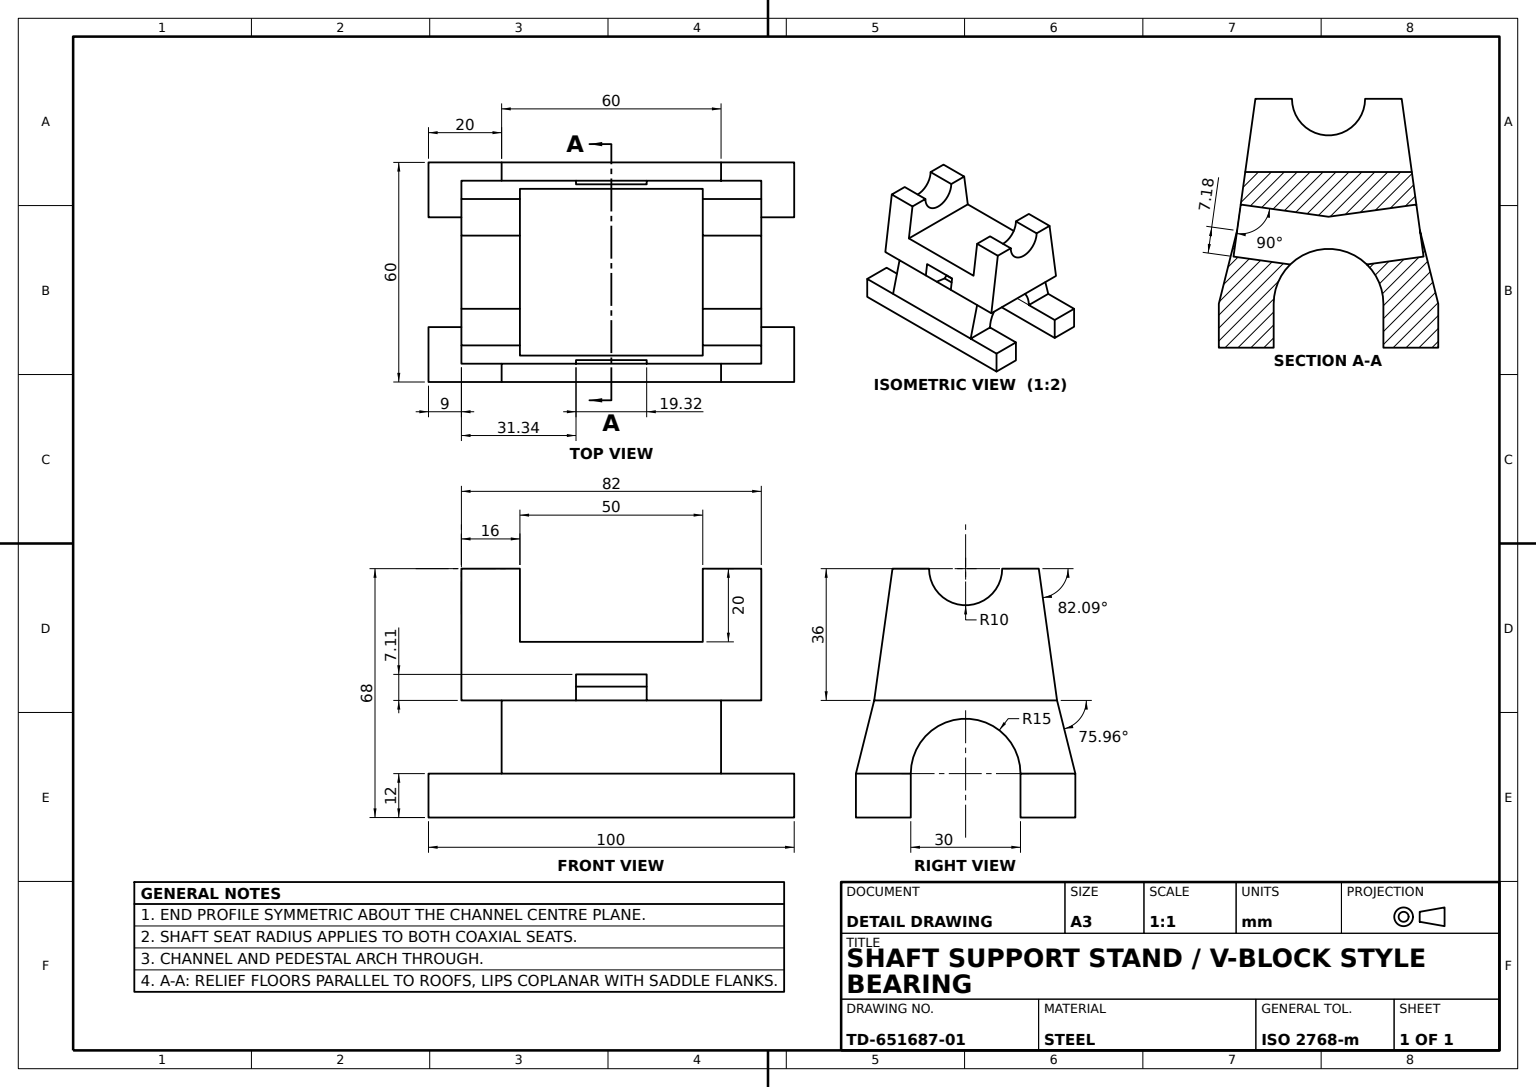
ISO-10303-21;
HEADER;
FILE_DESCRIPTION((''),'2;1');
FILE_NAME('','',(''),(''),'','','');
FILE_SCHEMA(('AUTOMOTIVE_DESIGN'));
ENDSEC;
DATA;
#1=APPLICATION_CONTEXT('');
#2=PRODUCT_CONTEXT('',#1,'mechanical');
#3=PRODUCT('','','',(#2));
#4=PRODUCT_DEFINITION_FORMATION('','',#3);
#5=PRODUCT_DEFINITION_CONTEXT('',#1,'design');
#6=PRODUCT_DEFINITION('','',#4,#5);
#7=PRODUCT_DEFINITION_SHAPE('','',#6);
#8=(LENGTH_UNIT()NAMED_UNIT(*)SI_UNIT(.MILLI.,.METRE.));
#9=(NAMED_UNIT(*)PLANE_ANGLE_UNIT()SI_UNIT($,.RADIAN.));
#10=(NAMED_UNIT(*)SI_UNIT($,.STERADIAN.)SOLID_ANGLE_UNIT());
#11=UNCERTAINTY_MEASURE_WITH_UNIT(LENGTH_MEASURE(1.E-05),#8,'distance_accuracy_value','');
#12=(GEOMETRIC_REPRESENTATION_CONTEXT(3)GLOBAL_UNCERTAINTY_ASSIGNED_CONTEXT((#11))GLOBAL_UNIT_ASSIGNED_CONTEXT((#8,#9,#10))REPRESENTATION_CONTEXT('',''));
#13=CARTESIAN_POINT('',(-15.,0.,-100.));
#14=VERTEX_POINT('',#13);
#15=CARTESIAN_POINT('',(-15.,0.,0.));
#16=VERTEX_POINT('',#15);
#17=DIRECTION('',(0.,0.,1.));
#18=VECTOR('',#17,1000.);
#19=LINE('',#15,#18);
#20=EDGE_CURVE('',#14,#16,#19,.T.);
#21=ORIENTED_EDGE('',*,*,#20,.T.);
#22=CARTESIAN_POINT('',(-30.,0.,0.));
#23=VERTEX_POINT('',#22);
#24=CARTESIAN_POINT('',(0.,0.,0.));
#25=DIRECTION('',(1.,0.,0.));
#26=VECTOR('',#25,1000.);
#27=LINE('',#24,#26);
#28=EDGE_CURVE('',#23,#16,#27,.T.);
#29=ORIENTED_EDGE('',*,*,#28,.F.);
#30=CARTESIAN_POINT('',(-30.,0.,-100.));
#31=VERTEX_POINT('',#30);
#32=LINE('',#30,#18);
#33=EDGE_CURVE('',#31,#23,#32,.T.);
#34=ORIENTED_EDGE('',*,*,#33,.F.);
#35=CARTESIAN_POINT('',(30.,0.,-100.));
#36=DIRECTION('',(-1.,0.,0.));
#37=VECTOR('',#36,1000.);
#38=LINE('',#35,#37);
#39=EDGE_CURVE('',#14,#31,#38,.T.);
#40=ORIENTED_EDGE('',*,*,#39,.F.);
#41=EDGE_LOOP('',(#21,#29,#34,#40));
#42=FACE_OUTER_BOUND('',#41,.T.);
#43=DIRECTION('',(0.,1.,0.));
#44=AXIS2_PLACEMENT_3D('',#24,#43,#17);
#45=PLANE('',#44);
#46=ADVANCED_FACE('',(#42),#45,.F.);
#47=CARTESIAN_POINT('',(-25.,32.,-80.));
#48=VERTEX_POINT('',#47);
#49=CARTESIAN_POINT('',(-30.,12.,-80.));
#50=VERTEX_POINT('',#49);
#51=DIRECTION('',(-0.242535625,-0.9701425,0.));
#52=VECTOR('',#51,1000.);
#53=LINE('',#47,#52);
#54=EDGE_CURVE('',#48,#50,#53,.T.);
#55=ORIENTED_EDGE('',*,*,#54,.T.);
#56=CARTESIAN_POINT('',(-30.,12.,-20.));
#57=VERTEX_POINT('',#56);
#58=LINE('',#49,#18);
#59=EDGE_CURVE('',#50,#57,#58,.T.);
#60=ORIENTED_EDGE('',*,*,#59,.T.);
#61=CARTESIAN_POINT('',(-25.,32.,-20.));
#62=VERTEX_POINT('',#61);
#63=LINE('',#61,#52);
#64=EDGE_CURVE('',#62,#57,#63,.T.);
#65=ORIENTED_EDGE('',*,*,#64,.F.);
#66=CARTESIAN_POINT('',(-25.,32.,-40.337526));
#67=VERTEX_POINT('',#66);
#68=LINE('',#47,#18);
#69=EDGE_CURVE('',#67,#62,#68,.T.);
#70=ORIENTED_EDGE('',*,*,#69,.F.);
#71=CARTESIAN_POINT('',(-25.,32.,-59.662474));
#72=VERTEX_POINT('',#71);
#73=EDGE_CURVE('',#72,#67,#68,.T.);
#74=ORIENTED_EDGE('',*,*,#73,.F.);
#75=EDGE_CURVE('',#48,#72,#68,.T.);
#76=ORIENTED_EDGE('',*,*,#75,.F.);
#77=EDGE_LOOP('',(#55,#60,#65,#70,#74,#76));
#78=FACE_OUTER_BOUND('',#77,.T.);
#79=DIRECTION('',(-0.9701425,0.242535625,0.));
#80=AXIS2_PLACEMENT_3D('',#47,#79,#51);
#81=PLANE('',#80);
#82=ADVANCED_FACE('',(#78),#81,.T.);
#83=CARTESIAN_POINT('',(-30.,12.,0.));
#84=VERTEX_POINT('',#83);
#85=CARTESIAN_POINT('',(-15.,12.,0.));
#86=VERTEX_POINT('',#85);
#87=LINE('',#83,#26);
#88=EDGE_CURVE('',#84,#86,#87,.T.);
#89=ORIENTED_EDGE('',*,*,#88,.T.);
#90=CARTESIAN_POINT('',(-15.,12.,-20.));
#91=VERTEX_POINT('',#90);
#92=CARTESIAN_POINT('',(-15.,12.,-100.));
#93=LINE('',#92,#18);
#94=EDGE_CURVE('',#91,#86,#93,.T.);
#95=ORIENTED_EDGE('',*,*,#94,.F.);
#96=LINE('',#56,#26);
#97=EDGE_CURVE('',#57,#91,#96,.T.);
#98=ORIENTED_EDGE('',*,*,#97,.F.);
#99=CARTESIAN_POINT('',(-30.,12.,-100.));
#100=LINE('',#99,#18);
#101=EDGE_CURVE('',#57,#84,#100,.T.);
#102=ORIENTED_EDGE('',*,*,#101,.T.);
#103=EDGE_LOOP('',(#89,#95,#98,#102));
#104=FACE_OUTER_BOUND('',#103,.T.);
#105=CARTESIAN_POINT('',(0.,12.,0.));
#106=AXIS2_PLACEMENT_3D('',#105,#43,#17);
#107=PLANE('',#106);
#108=ADVANCED_FACE('',(#104),#107,.T.);
#109=CARTESIAN_POINT('',(-10.,68.,-75.));
#110=VERTEX_POINT('',#109);
#111=CARTESIAN_POINT('',(-20.,68.,-75.));
#112=VERTEX_POINT('',#111);
#113=LINE('',#111,#37);
#114=EDGE_CURVE('',#110,#112,#113,.T.);
#115=ORIENTED_EDGE('',*,*,#114,.T.);
#116=CARTESIAN_POINT('',(-22.777778,48.,-75.));
#117=VERTEX_POINT('',#116);
#118=DIRECTION('',(-0.137568371,-0.990492273,0.));
#119=VECTOR('',#118,1000.);
#120=LINE('',#111,#119);
#121=EDGE_CURVE('',#112,#117,#120,.T.);
#122=ORIENTED_EDGE('',*,*,#121,.T.);
#123=CARTESIAN_POINT('',(22.777778,48.,-75.));
#124=VERTEX_POINT('',#123);
#125=CARTESIAN_POINT('',(20.,48.,-75.));
#126=LINE('',#125,#37);
#127=EDGE_CURVE('',#124,#117,#126,.T.);
#128=ORIENTED_EDGE('',*,*,#127,.F.);
#129=CARTESIAN_POINT('',(20.,68.,-75.));
#130=VERTEX_POINT('',#129);
#131=DIRECTION('',(-0.137568371,0.990492273,0.));
#132=VECTOR('',#131,1000.);
#133=LINE('',#129,#132);
#134=EDGE_CURVE('',#124,#130,#133,.T.);
#135=ORIENTED_EDGE('',*,*,#134,.T.);
#136=CARTESIAN_POINT('',(10.,68.,-75.));
#137=VERTEX_POINT('',#136);
#138=EDGE_CURVE('',#130,#137,#113,.T.);
#139=ORIENTED_EDGE('',*,*,#138,.T.);
#140=CARTESIAN_POINT('',(0.,68.,-75.));
#141=DIRECTION('',(0.,0.,-1.));
#142=AXIS2_PLACEMENT_3D('',#140,#141,#36);
#143=CIRCLE('',#142,10.);
#144=EDGE_CURVE('',#137,#110,#143,.T.);
#145=ORIENTED_EDGE('',*,*,#144,.T.);
#146=EDGE_LOOP('',(#115,#122,#128,#135,#139,#145));
#147=FACE_OUTER_BOUND('',#146,.T.);
#148=CARTESIAN_POINT('',(-20.,48.,-75.));
#149=AXIS2_PLACEMENT_3D('',#148,#141,#36);
#150=PLANE('',#149);
#151=ADVANCED_FACE('',(#147),#150,.F.);
#152=CARTESIAN_POINT('',(-25.987343,24.891129,-59.662474));
#153=VERTEX_POINT('',#152);
#154=DIRECTION('',(0.137568371,0.990492273,0.));
#155=VECTOR('',#154,1000.);
#156=LINE('',#152,#155);
#157=EDGE_CURVE('',#153,#72,#156,.T.);
#158=ORIENTED_EDGE('',*,*,#157,.F.);
#159=CARTESIAN_POINT('',(-10.474958,22.736632,-59.662474));
#160=VERTEX_POINT('',#159);
#161=CARTESIAN_POINT('',(1.746441,21.039215,-59.662474));
#162=DIRECTION('',(-0.990492273,0.137568371,0.));
#163=VECTOR('',#162,1000.);
#164=LINE('',#161,#163);
#165=EDGE_CURVE('',#160,#153,#164,.T.);
#166=ORIENTED_EDGE('',*,*,#165,.F.);
#167=CARTESIAN_POINT('',(10.474958,22.736632,-59.662474));
#168=VERTEX_POINT('',#167);
#169=CARTESIAN_POINT('',(0.,12.,-59.662474));
#170=AXIS2_PLACEMENT_3D('',#169,#141,#36);
#171=CIRCLE('',#170,15.);
#172=EDGE_CURVE('',#160,#168,#171,.T.);
#173=ORIENTED_EDGE('',*,*,#172,.T.);
#174=CARTESIAN_POINT('',(25.987343,24.891129,-59.662474));
#175=VERTEX_POINT('',#174);
#176=CARTESIAN_POINT('',(-1.746441,21.039215,-59.662474));
#177=DIRECTION('',(0.990492273,0.137568371,0.));
#178=VECTOR('',#177,1000.);
#179=LINE('',#176,#178);
#180=EDGE_CURVE('',#168,#175,#179,.T.);
#181=ORIENTED_EDGE('',*,*,#180,.T.);
#182=CARTESIAN_POINT('',(25.,32.,-59.662474));
#183=VERTEX_POINT('',#182);
#184=LINE('',#174,#132);
#185=EDGE_CURVE('',#175,#183,#184,.T.);
#186=ORIENTED_EDGE('',*,*,#185,.T.);
#187=CARTESIAN_POINT('',(24.012657,39.108871,-59.662474));
#188=VERTEX_POINT('',#187);
#189=CARTESIAN_POINT('',(20.,68.,-59.662474));
#190=LINE('',#189,#132);
#191=EDGE_CURVE('',#183,#188,#190,.T.);
#192=ORIENTED_EDGE('',*,*,#191,.T.);
#193=CARTESIAN_POINT('',(0.,35.773779,-59.662474));
#194=VERTEX_POINT('',#193);
#195=CARTESIAN_POINT('',(-3.721127,35.256956,-59.662474));
#196=LINE('',#195,#178);
#197=EDGE_CURVE('',#194,#188,#196,.T.);
#198=ORIENTED_EDGE('',*,*,#197,.F.);
#199=CARTESIAN_POINT('',(-24.012657,39.108871,-59.662474));
#200=VERTEX_POINT('',#199);
#201=CARTESIAN_POINT('',(3.721127,35.256956,-59.662474));
#202=LINE('',#201,#163);
#203=EDGE_CURVE('',#194,#200,#202,.T.);
#204=ORIENTED_EDGE('',*,*,#203,.T.);
#205=EDGE_CURVE('',#72,#200,#156,.T.);
#206=ORIENTED_EDGE('',*,*,#205,.F.);
#207=EDGE_LOOP('',(#158,#166,#173,#181,#186,#192,#198,#204,#206));
#208=FACE_OUTER_BOUND('',#207,.T.);
#209=AXIS2_PLACEMENT_3D('',#176,#141,#36);
#210=PLANE('',#209);
#211=ADVANCED_FACE('',(#208),#210,.F.);
#212=VERTEX_POINT('',#92);
#213=CARTESIAN_POINT('',(-15.,-61.,-100.));
#214=VECTOR('',#43,1000.);
#215=LINE('',#213,#214);
#216=EDGE_CURVE('',#14,#212,#215,.T.);
#217=ORIENTED_EDGE('',*,*,#216,.F.);
#218=ORIENTED_EDGE('',*,*,#39,.T.);
#219=VERTEX_POINT('',#99);
#220=DIRECTION('',(0.,-1.,0.));
#221=VECTOR('',#220,1000.);
#222=LINE('',#99,#221);
#223=EDGE_CURVE('',#219,#31,#222,.T.);
#224=ORIENTED_EDGE('',*,*,#223,.F.);
#225=CARTESIAN_POINT('',(30.,12.,-100.));
#226=LINE('',#225,#37);
#227=EDGE_CURVE('',#212,#219,#226,.T.);
#228=ORIENTED_EDGE('',*,*,#227,.F.);
#229=EDGE_LOOP('',(#217,#218,#224,#228));
#230=FACE_OUTER_BOUND('',#229,.T.);
#231=AXIS2_PLACEMENT_3D('',#225,#17,#25);
#232=PLANE('',#231);
#233=ADVANCED_FACE('',(#230),#232,.F.);
#234=ORIENTED_EDGE('',*,*,#69,.T.);
#235=CARTESIAN_POINT('',(-25.,32.,-9.));
#236=VERTEX_POINT('',#235);
#237=CARTESIAN_POINT('',(-25.,32.,-91.));
#238=LINE('',#237,#18);
#239=EDGE_CURVE('',#62,#236,#238,.T.);
#240=ORIENTED_EDGE('',*,*,#239,.T.);
#241=CARTESIAN_POINT('',(-20.,68.,-9.));
#242=VERTEX_POINT('',#241);
#243=LINE('',#241,#119);
#244=EDGE_CURVE('',#242,#236,#243,.T.);
#245=ORIENTED_EDGE('',*,*,#244,.F.);
#246=CARTESIAN_POINT('',(-20.,68.,-25.));
#247=VERTEX_POINT('',#246);
#248=CARTESIAN_POINT('',(-20.,68.,-91.));
#249=LINE('',#248,#18);
#250=EDGE_CURVE('',#247,#242,#249,.T.);
#251=ORIENTED_EDGE('',*,*,#250,.F.);
#252=CARTESIAN_POINT('',(-22.777778,48.,-25.));
#253=VERTEX_POINT('',#252);
#254=LINE('',#246,#155);
#255=EDGE_CURVE('',#253,#247,#254,.T.);
#256=ORIENTED_EDGE('',*,*,#255,.F.);
#257=CARTESIAN_POINT('',(-22.777778,48.,-91.));
#258=LINE('',#257,#18);
#259=EDGE_CURVE('',#117,#253,#258,.T.);
#260=ORIENTED_EDGE('',*,*,#259,.F.);
#261=ORIENTED_EDGE('',*,*,#121,.F.);
#262=VERTEX_POINT('',#248);
#263=EDGE_CURVE('',#262,#112,#249,.T.);
#264=ORIENTED_EDGE('',*,*,#263,.F.);
#265=VERTEX_POINT('',#237);
#266=LINE('',#248,#119);
#267=EDGE_CURVE('',#262,#265,#266,.T.);
#268=ORIENTED_EDGE('',*,*,#267,.T.);
#269=EDGE_CURVE('',#265,#48,#238,.T.);
#270=ORIENTED_EDGE('',*,*,#269,.T.);
#271=ORIENTED_EDGE('',*,*,#75,.T.);
#272=ORIENTED_EDGE('',*,*,#205,.T.);
#273=CARTESIAN_POINT('',(-24.012657,39.108871,-40.337526));
#274=VERTEX_POINT('',#273);
#275=LINE('',#273,#18);
#276=EDGE_CURVE('',#200,#274,#275,.T.);
#277=ORIENTED_EDGE('',*,*,#276,.T.);
#278=CARTESIAN_POINT('',(-25.987343,24.891129,-40.337526));
#279=LINE('',#278,#119);
#280=EDGE_CURVE('',#274,#67,#279,.T.);
#281=ORIENTED_EDGE('',*,*,#280,.T.);
#282=EDGE_LOOP('',(#234,#240,#245,#251,#256,#260,#261,#264,#268,#270,#271,#272,#277,#281));
#283=FACE_OUTER_BOUND('',#282,.T.);
#284=AXIS2_PLACEMENT_3D('',#248,#162,#118);
#285=PLANE('',#284);
#286=ADVANCED_FACE('',(#283),#285,.T.);
#287=CARTESIAN_POINT('',(10.,68.,-9.));
#288=VERTEX_POINT('',#287);
#289=CARTESIAN_POINT('',(-10.,68.,-9.));
#290=VERTEX_POINT('',#289);
#291=CARTESIAN_POINT('',(0.,68.,-9.));
#292=AXIS2_PLACEMENT_3D('',#291,#141,#25);
#293=CIRCLE('',#292,10.);
#294=EDGE_CURVE('',#288,#290,#293,.T.);
#295=ORIENTED_EDGE('',*,*,#294,.T.);
#296=LINE('',#289,#37);
#297=EDGE_CURVE('',#290,#242,#296,.T.);
#298=ORIENTED_EDGE('',*,*,#297,.T.);
#299=ORIENTED_EDGE('',*,*,#244,.T.);
#300=CARTESIAN_POINT('',(25.,32.,-9.));
#301=VERTEX_POINT('',#300);
#302=LINE('',#235,#26);
#303=EDGE_CURVE('',#236,#301,#302,.T.);
#304=ORIENTED_EDGE('',*,*,#303,.T.);
#305=CARTESIAN_POINT('',(20.,68.,-9.));
#306=VERTEX_POINT('',#305);
#307=LINE('',#305,#132);
#308=EDGE_CURVE('',#301,#306,#307,.T.);
#309=ORIENTED_EDGE('',*,*,#308,.T.);
#310=LINE('',#287,#37);
#311=EDGE_CURVE('',#306,#288,#310,.T.);
#312=ORIENTED_EDGE('',*,*,#311,.T.);
#313=EDGE_LOOP('',(#295,#298,#299,#304,#309,#312));
#314=FACE_OUTER_BOUND('',#313,.T.);
#315=AXIS2_PLACEMENT_3D('',#291,#17,#25);
#316=PLANE('',#315);
#317=ADVANCED_FACE('',(#314),#316,.T.);
#318=CARTESIAN_POINT('',(-15.,-61.,0.));
#319=LINE('',#318,#214);
#320=EDGE_CURVE('',#16,#86,#319,.T.);
#321=ORIENTED_EDGE('',*,*,#320,.F.);
#322=ORIENTED_EDGE('',*,*,#20,.F.);
#323=ORIENTED_EDGE('',*,*,#216,.T.);
#324=CARTESIAN_POINT('',(-15.,12.,-80.));
#325=VERTEX_POINT('',#324);
#326=EDGE_CURVE('',#212,#325,#93,.T.);
#327=ORIENTED_EDGE('',*,*,#326,.T.);
#328=LINE('',#324,#18);
#329=EDGE_CURVE('',#325,#91,#328,.T.);
#330=ORIENTED_EDGE('',*,*,#329,.T.);
#331=ORIENTED_EDGE('',*,*,#94,.T.);
#332=EDGE_LOOP('',(#321,#322,#323,#327,#330,#331));
#333=FACE_OUTER_BOUND('',#332,.T.);
#334=AXIS2_PLACEMENT_3D('',#213,#36,#17);
#335=PLANE('',#334);
#336=ADVANCED_FACE('',(#333),#335,.F.);
#337=ORIENTED_EDGE('',*,*,#263,.T.);
#338=ORIENTED_EDGE('',*,*,#114,.F.);
#339=CARTESIAN_POINT('',(-10.,68.,-91.));
#340=VERTEX_POINT('',#339);
#341=LINE('',#339,#18);
#342=EDGE_CURVE('',#340,#110,#341,.T.);
#343=ORIENTED_EDGE('',*,*,#342,.F.);
#344=LINE('',#339,#37);
#345=EDGE_CURVE('',#340,#262,#344,.T.);
#346=ORIENTED_EDGE('',*,*,#345,.T.);
#347=EDGE_LOOP('',(#337,#338,#343,#346));
#348=FACE_OUTER_BOUND('',#347,.T.);
#349=AXIS2_PLACEMENT_3D('',#339,#43,#17);
#350=PLANE('',#349);
#351=ADVANCED_FACE('',(#348),#350,.T.);
#352=CARTESIAN_POINT('',(10.474958,22.736632,-40.337526));
#353=VERTEX_POINT('',#352);
#354=CARTESIAN_POINT('',(10.474958,22.736632,-80.));
#355=LINE('',#354,#18);
#356=EDGE_CURVE('',#168,#353,#355,.T.);
#357=ORIENTED_EDGE('',*,*,#356,.F.);
#358=ORIENTED_EDGE('',*,*,#172,.F.);
#359=CARTESIAN_POINT('',(-10.474958,22.736632,-40.337526));
#360=VERTEX_POINT('',#359);
#361=CARTESIAN_POINT('',(-10.474958,22.736632,-80.));
#362=LINE('',#361,#18);
#363=EDGE_CURVE('',#160,#360,#362,.T.);
#364=ORIENTED_EDGE('',*,*,#363,.T.);
#365=CARTESIAN_POINT('',(0.,12.,-40.337526));
#366=AXIS2_PLACEMENT_3D('',#365,#17,#25);
#367=CIRCLE('',#366,15.);
#368=EDGE_CURVE('',#353,#360,#367,.T.);
#369=ORIENTED_EDGE('',*,*,#368,.F.);
#370=EDGE_LOOP('',(#357,#358,#364,#369));
#371=FACE_BOUND('',#370,.T.);
#372=CARTESIAN_POINT('',(15.,12.,-20.));
#373=VERTEX_POINT('',#372);
#374=CARTESIAN_POINT('',(0.,12.,-20.));
#375=AXIS2_PLACEMENT_3D('',#374,#141,#25);
#376=CIRCLE('',#375,15.);
#377=EDGE_CURVE('',#91,#373,#376,.T.);
#378=ORIENTED_EDGE('',*,*,#377,.F.);
#379=ORIENTED_EDGE('',*,*,#329,.F.);
#380=CARTESIAN_POINT('',(15.,12.,-80.));
#381=VERTEX_POINT('',#380);
#382=CARTESIAN_POINT('',(0.,12.,-80.));
#383=AXIS2_PLACEMENT_3D('',#382,#141,#25);
#384=CIRCLE('',#383,15.);
#385=EDGE_CURVE('',#325,#381,#384,.T.);
#386=ORIENTED_EDGE('',*,*,#385,.T.);
#387=LINE('',#380,#18);
#388=EDGE_CURVE('',#381,#373,#387,.T.);
#389=ORIENTED_EDGE('',*,*,#388,.T.);
#390=EDGE_LOOP('',(#378,#379,#386,#389));
#391=FACE_OUTER_BOUND('',#390,.T.);
#392=AXIS2_PLACEMENT_3D('',#382,#17,#25);
#393=CYLINDRICAL_SURFACE('',#392,15.);
#394=ADVANCED_FACE('',(#371,#391),#393,.F.);
#395=ORIENTED_EDGE('',*,*,#388,.F.);
#396=CARTESIAN_POINT('',(15.,12.,-100.));
#397=VERTEX_POINT('',#396);
#398=CARTESIAN_POINT('',(15.,12.,0.));
#399=VECTOR('',#141,1000.);
#400=LINE('',#398,#399);
#401=EDGE_CURVE('',#381,#397,#400,.T.);
#402=ORIENTED_EDGE('',*,*,#401,.T.);
#403=CARTESIAN_POINT('',(15.,0.,-100.));
#404=VERTEX_POINT('',#403);
#405=CARTESIAN_POINT('',(15.,-61.,-100.));
#406=LINE('',#405,#214);
#407=EDGE_CURVE('',#404,#397,#406,.T.);
#408=ORIENTED_EDGE('',*,*,#407,.F.);
#409=CARTESIAN_POINT('',(15.,0.,0.));
#410=VERTEX_POINT('',#409);
#411=LINE('',#409,#399);
#412=EDGE_CURVE('',#410,#404,#411,.T.);
#413=ORIENTED_EDGE('',*,*,#412,.F.);
#414=VERTEX_POINT('',#398);
#415=CARTESIAN_POINT('',(15.,-61.,0.));
#416=LINE('',#415,#214);
#417=EDGE_CURVE('',#410,#414,#416,.T.);
#418=ORIENTED_EDGE('',*,*,#417,.T.);
#419=EDGE_CURVE('',#414,#373,#400,.T.);
#420=ORIENTED_EDGE('',*,*,#419,.T.);
#421=EDGE_LOOP('',(#395,#402,#408,#413,#418,#420));
#422=FACE_OUTER_BOUND('',#421,.T.);
#423=AXIS2_PLACEMENT_3D('',#415,#25,#141);
#424=PLANE('',#423);
#425=ADVANCED_FACE('',(#422),#424,.F.);
#426=VERTEX_POINT('',#225);
#427=VERTEX_POINT('',#35);
#428=LINE('',#225,#221);
#429=EDGE_CURVE('',#426,#427,#428,.T.);
#430=ORIENTED_EDGE('',*,*,#429,.T.);
#431=EDGE_CURVE('',#427,#404,#38,.T.);
#432=ORIENTED_EDGE('',*,*,#431,.T.);
#433=ORIENTED_EDGE('',*,*,#407,.T.);
#434=EDGE_CURVE('',#426,#397,#226,.T.);
#435=ORIENTED_EDGE('',*,*,#434,.F.);
#436=EDGE_LOOP('',(#430,#432,#433,#435));
#437=FACE_OUTER_BOUND('',#436,.T.);
#438=ADVANCED_FACE('',(#437),#232,.F.);
#439=ORIENTED_EDGE('',*,*,#276,.F.);
#440=ORIENTED_EDGE('',*,*,#203,.F.);
#441=CARTESIAN_POINT('',(0.,35.773779,-40.337526));
#442=VERTEX_POINT('',#441);
#443=LINE('',#441,#18);
#444=EDGE_CURVE('',#194,#442,#443,.T.);
#445=ORIENTED_EDGE('',*,*,#444,.T.);
#446=CARTESIAN_POINT('',(3.721127,35.256956,-40.337526));
#447=LINE('',#446,#163);
#448=EDGE_CURVE('',#442,#274,#447,.T.);
#449=ORIENTED_EDGE('',*,*,#448,.T.);
#450=EDGE_LOOP('',(#439,#440,#445,#449));
#451=FACE_OUTER_BOUND('',#450,.T.);
#452=DIRECTION('',(0.990492273,-0.137568371,0.));
#453=AXIS2_PLACEMENT_3D('',#446,#118,#452);
#454=PLANE('',#453);
#455=ADVANCED_FACE('',(#451),#454,.T.);
#456=ORIENTED_EDGE('',*,*,#401,.F.);
#457=CARTESIAN_POINT('',(30.,12.,-80.));
#458=VERTEX_POINT('',#457);
#459=LINE('',#380,#26);
#460=EDGE_CURVE('',#381,#458,#459,.T.);
#461=ORIENTED_EDGE('',*,*,#460,.T.);
#462=CARTESIAN_POINT('',(30.,12.,0.));
#463=LINE('',#462,#399);
#464=EDGE_CURVE('',#458,#426,#463,.T.);
#465=ORIENTED_EDGE('',*,*,#464,.T.);
#466=ORIENTED_EDGE('',*,*,#434,.T.);
#467=EDGE_LOOP('',(#456,#461,#465,#466));
#468=FACE_OUTER_BOUND('',#467,.T.);
#469=ADVANCED_FACE('',(#468),#107,.T.);
#470=ORIENTED_EDGE('',*,*,#280,.F.);
#471=ORIENTED_EDGE('',*,*,#448,.F.);
#472=CARTESIAN_POINT('',(24.012657,39.108871,-40.337526));
#473=VERTEX_POINT('',#472);
#474=CARTESIAN_POINT('',(-3.721127,35.256956,-40.337526));
#475=LINE('',#474,#178);
#476=EDGE_CURVE('',#442,#473,#475,.T.);
#477=ORIENTED_EDGE('',*,*,#476,.T.);
#478=CARTESIAN_POINT('',(25.,32.,-40.337526));
#479=VERTEX_POINT('',#478);
#480=CARTESIAN_POINT('',(25.987343,24.891129,-40.337526));
#481=DIRECTION('',(0.137568371,-0.990492273,0.));
#482=VECTOR('',#481,1000.);
#483=LINE('',#480,#482);
#484=EDGE_CURVE('',#473,#479,#483,.T.);
#485=ORIENTED_EDGE('',*,*,#484,.T.);
#486=VERTEX_POINT('',#480);
#487=EDGE_CURVE('',#479,#486,#483,.T.);
#488=ORIENTED_EDGE('',*,*,#487,.T.);
#489=CARTESIAN_POINT('',(-1.746441,21.039215,-40.337526));
#490=LINE('',#489,#178);
#491=EDGE_CURVE('',#353,#486,#490,.T.);
#492=ORIENTED_EDGE('',*,*,#491,.F.);
#493=ORIENTED_EDGE('',*,*,#368,.T.);
#494=VERTEX_POINT('',#278);
#495=CARTESIAN_POINT('',(1.746441,21.039215,-40.337526));
#496=LINE('',#495,#163);
#497=EDGE_CURVE('',#360,#494,#496,.T.);
#498=ORIENTED_EDGE('',*,*,#497,.T.);
#499=EDGE_CURVE('',#67,#494,#279,.T.);
#500=ORIENTED_EDGE('',*,*,#499,.F.);
#501=EDGE_LOOP('',(#470,#471,#477,#485,#488,#492,#493,#498,#500));
#502=FACE_OUTER_BOUND('',#501,.T.);
#503=AXIS2_PLACEMENT_3D('',#489,#17,#25);
#504=PLANE('',#503);
#505=ADVANCED_FACE('',(#502),#504,.F.);
#506=ORIENTED_EDGE('',*,*,#303,.F.);
#507=ORIENTED_EDGE('',*,*,#239,.F.);
#508=CARTESIAN_POINT('',(25.,32.,-20.));
#509=VERTEX_POINT('',#508);
#510=CARTESIAN_POINT('',(0.,32.,-20.));
#511=LINE('',#510,#37);
#512=EDGE_CURVE('',#509,#62,#511,.T.);
#513=ORIENTED_EDGE('',*,*,#512,.F.);
#514=CARTESIAN_POINT('',(25.,32.,-91.));
#515=LINE('',#514,#18);
#516=EDGE_CURVE('',#509,#301,#515,.T.);
#517=ORIENTED_EDGE('',*,*,#516,.T.);
#518=EDGE_LOOP('',(#506,#507,#513,#517));
#519=FACE_OUTER_BOUND('',#518,.T.);
#520=AXIS2_PLACEMENT_3D('',#237,#220,#141);
#521=PLANE('',#520);
#522=ADVANCED_FACE('',(#519),#521,.T.);
#523=CARTESIAN_POINT('',(10.,68.,-25.));
#524=VERTEX_POINT('',#523);
#525=CARTESIAN_POINT('',(20.,68.,-25.));
#526=VERTEX_POINT('',#525);
#527=CARTESIAN_POINT('',(26.893268,68.,-25.));
#528=LINE('',#527,#26);
#529=EDGE_CURVE('',#524,#526,#528,.T.);
#530=ORIENTED_EDGE('',*,*,#529,.F.);
#531=CARTESIAN_POINT('',(10.,68.,-91.));
#532=LINE('',#531,#18);
#533=EDGE_CURVE('',#524,#288,#532,.T.);
#534=ORIENTED_EDGE('',*,*,#533,.T.);
#535=ORIENTED_EDGE('',*,*,#311,.F.);
#536=CARTESIAN_POINT('',(20.,68.,-91.));
#537=LINE('',#536,#18);
#538=EDGE_CURVE('',#526,#306,#537,.T.);
#539=ORIENTED_EDGE('',*,*,#538,.F.);
#540=EDGE_LOOP('',(#530,#534,#535,#539));
#541=FACE_OUTER_BOUND('',#540,.T.);
#542=AXIS2_PLACEMENT_3D('',#531,#43,#17);
#543=PLANE('',#542);
#544=ADVANCED_FACE('',(#541),#543,.T.);
#545=VERTEX_POINT('',#514);
#546=VERTEX_POINT('',#536);
#547=LINE('',#536,#132);
#548=EDGE_CURVE('',#545,#546,#547,.T.);
#549=ORIENTED_EDGE('',*,*,#548,.F.);
#550=LINE('',#514,#26);
#551=EDGE_CURVE('',#265,#545,#550,.T.);
#552=ORIENTED_EDGE('',*,*,#551,.F.);
#553=ORIENTED_EDGE('',*,*,#267,.F.);
#554=ORIENTED_EDGE('',*,*,#345,.F.);
#555=VERTEX_POINT('',#531);
#556=CARTESIAN_POINT('',(0.,68.,-91.));
#557=AXIS2_PLACEMENT_3D('',#556,#141,#25);
#558=CIRCLE('',#557,10.);
#559=EDGE_CURVE('',#555,#340,#558,.T.);
#560=ORIENTED_EDGE('',*,*,#559,.F.);
#561=LINE('',#531,#37);
#562=EDGE_CURVE('',#546,#555,#561,.T.);
#563=ORIENTED_EDGE('',*,*,#562,.F.);
#564=EDGE_LOOP('',(#549,#552,#553,#554,#560,#563));
#565=FACE_OUTER_BOUND('',#564,.T.);
#566=AXIS2_PLACEMENT_3D('',#556,#17,#25);
#567=PLANE('',#566);
#568=ADVANCED_FACE('',(#565),#567,.F.);
#569=CARTESIAN_POINT('',(25.,32.,-80.));
#570=VERTEX_POINT('',#569);
#571=CARTESIAN_POINT('',(0.,32.,-80.));
#572=LINE('',#571,#37);
#573=EDGE_CURVE('',#570,#48,#572,.T.);
#574=ORIENTED_EDGE('',*,*,#573,.F.);
#575=DIRECTION('',(-0.242535625,0.9701425,0.));
#576=VECTOR('',#575,1000.);
#577=LINE('',#569,#576);
#578=EDGE_CURVE('',#458,#570,#577,.T.);
#579=ORIENTED_EDGE('',*,*,#578,.F.);
#580=ORIENTED_EDGE('',*,*,#460,.F.);
#581=ORIENTED_EDGE('',*,*,#385,.F.);
#582=LINE('',#49,#26);
#583=EDGE_CURVE('',#50,#325,#582,.T.);
#584=ORIENTED_EDGE('',*,*,#583,.F.);
#585=ORIENTED_EDGE('',*,*,#54,.F.);
#586=EDGE_LOOP('',(#574,#579,#580,#581,#584,#585));
#587=FACE_OUTER_BOUND('',#586,.T.);
#588=PLANE('',#392);
#589=ADVANCED_FACE('',(#587),#588,.F.);
#590=ORIENTED_EDGE('',*,*,#487,.F.);
#591=LINE('',#569,#18);
#592=EDGE_CURVE('',#183,#479,#591,.T.);
#593=ORIENTED_EDGE('',*,*,#592,.F.);
#594=ORIENTED_EDGE('',*,*,#185,.F.);
#595=LINE('',#480,#399);
#596=EDGE_CURVE('',#486,#175,#595,.T.);
#597=ORIENTED_EDGE('',*,*,#596,.F.);
#598=EDGE_LOOP('',(#590,#593,#594,#597));
#599=FACE_OUTER_BOUND('',#598,.T.);
#600=CARTESIAN_POINT('',(28.887207,4.012112,0.));
#601=DIRECTION('',(-0.990492273,-0.137568371,0.));
#602=AXIS2_PLACEMENT_3D('',#600,#601,#481);
#603=PLANE('',#602);
#604=ADVANCED_FACE('',(#599),#603,.T.);
#605=ORIENTED_EDGE('',*,*,#294,.F.);
#606=ORIENTED_EDGE('',*,*,#533,.F.);
#607=CARTESIAN_POINT('',(-10.,68.,-25.));
#608=VERTEX_POINT('',#607);
#609=CARTESIAN_POINT('',(0.,68.,-25.));
#610=AXIS2_PLACEMENT_3D('',#609,#17,#25);
#611=CIRCLE('',#610,10.);
#612=EDGE_CURVE('',#608,#524,#611,.T.);
#613=ORIENTED_EDGE('',*,*,#612,.F.);
#614=EDGE_CURVE('',#608,#290,#341,.T.);
#615=ORIENTED_EDGE('',*,*,#614,.T.);
#616=EDGE_LOOP('',(#605,#606,#613,#615));
#617=FACE_OUTER_BOUND('',#616,.T.);
#618=CYLINDRICAL_SURFACE('',#566,10.);
#619=ADVANCED_FACE('',(#617),#618,.F.);
#620=VERTEX_POINT('',#462);
#621=CARTESIAN_POINT('',(30.,12.,-20.));
#622=VERTEX_POINT('',#621);
#623=EDGE_CURVE('',#620,#622,#463,.T.);
#624=ORIENTED_EDGE('',*,*,#623,.T.);
#625=LINE('',#372,#26);
#626=EDGE_CURVE('',#373,#622,#625,.T.);
#627=ORIENTED_EDGE('',*,*,#626,.F.);
#628=ORIENTED_EDGE('',*,*,#419,.F.);
#629=EDGE_CURVE('',#414,#620,#87,.T.);
#630=ORIENTED_EDGE('',*,*,#629,.T.);
#631=EDGE_LOOP('',(#624,#627,#628,#630));
#632=FACE_OUTER_BOUND('',#631,.T.);
#633=ADVANCED_FACE('',(#632),#107,.T.);
#634=EDGE_CURVE('',#219,#50,#100,.T.);
#635=ORIENTED_EDGE('',*,*,#634,.T.);
#636=ORIENTED_EDGE('',*,*,#583,.T.);
#637=ORIENTED_EDGE('',*,*,#326,.F.);
#638=ORIENTED_EDGE('',*,*,#227,.T.);
#639=EDGE_LOOP('',(#635,#636,#637,#638));
#640=FACE_OUTER_BOUND('',#639,.T.);
#641=ADVANCED_FACE('',(#640),#107,.T.);
#642=ORIENTED_EDGE('',*,*,#634,.F.);
#643=ORIENTED_EDGE('',*,*,#223,.T.);
#644=ORIENTED_EDGE('',*,*,#33,.T.);
#645=LINE('',#83,#221);
#646=EDGE_CURVE('',#84,#23,#645,.T.);
#647=ORIENTED_EDGE('',*,*,#646,.F.);
#648=ORIENTED_EDGE('',*,*,#101,.F.);
#649=ORIENTED_EDGE('',*,*,#59,.F.);
#650=EDGE_LOOP('',(#642,#643,#644,#647,#648,#649));
#651=FACE_OUTER_BOUND('',#650,.T.);
#652=AXIS2_PLACEMENT_3D('',#99,#25,#141);
#653=PLANE('',#652);
#654=ADVANCED_FACE('',(#651),#653,.F.);
#655=ORIENTED_EDGE('',*,*,#377,.T.);
#656=ORIENTED_EDGE('',*,*,#626,.T.);
#657=LINE('',#508,#576);
#658=EDGE_CURVE('',#622,#509,#657,.T.);
#659=ORIENTED_EDGE('',*,*,#658,.T.);
#660=ORIENTED_EDGE('',*,*,#512,.T.);
#661=ORIENTED_EDGE('',*,*,#64,.T.);
#662=ORIENTED_EDGE('',*,*,#97,.T.);
#663=EDGE_LOOP('',(#655,#656,#659,#660,#661,#662));
#664=FACE_OUTER_BOUND('',#663,.T.);
#665=AXIS2_PLACEMENT_3D('',#374,#17,#25);
#666=PLANE('',#665);
#667=ADVANCED_FACE('',(#664),#666,.T.);
#668=EDGE_CURVE('',#555,#137,#532,.T.);
#669=ORIENTED_EDGE('',*,*,#668,.T.);
#670=ORIENTED_EDGE('',*,*,#138,.F.);
#671=EDGE_CURVE('',#546,#130,#537,.T.);
#672=ORIENTED_EDGE('',*,*,#671,.F.);
#673=ORIENTED_EDGE('',*,*,#562,.T.);
#674=EDGE_LOOP('',(#669,#670,#672,#673));
#675=FACE_OUTER_BOUND('',#674,.T.);
#676=ADVANCED_FACE('',(#675),#543,.T.);
#677=EDGE_CURVE('',#247,#608,#528,.T.);
#678=ORIENTED_EDGE('',*,*,#677,.F.);
#679=ORIENTED_EDGE('',*,*,#250,.T.);
#680=ORIENTED_EDGE('',*,*,#297,.F.);
#681=ORIENTED_EDGE('',*,*,#614,.F.);
#682=EDGE_LOOP('',(#678,#679,#680,#681));
#683=FACE_OUTER_BOUND('',#682,.T.);
#684=ADVANCED_FACE('',(#683),#350,.T.);
#685=CARTESIAN_POINT('',(22.777778,48.,-25.));
#686=VERTEX_POINT('',#685);
#687=CARTESIAN_POINT('',(-29.513236,48.,-25.));
#688=LINE('',#687,#26);
#689=EDGE_CURVE('',#253,#686,#688,.T.);
#690=ORIENTED_EDGE('',*,*,#689,.T.);
#691=CARTESIAN_POINT('',(22.777778,48.,-91.));
#692=LINE('',#691,#399);
#693=EDGE_CURVE('',#686,#124,#692,.T.);
#694=ORIENTED_EDGE('',*,*,#693,.T.);
#695=ORIENTED_EDGE('',*,*,#127,.T.);
#696=ORIENTED_EDGE('',*,*,#259,.T.);
#697=EDGE_LOOP('',(#690,#694,#695,#696));
#698=FACE_OUTER_BOUND('',#697,.T.);
#699=CARTESIAN_POINT('',(0.,48.,0.));
#700=AXIS2_PLACEMENT_3D('',#699,#220,#141);
#701=PLANE('',#700);
#702=ADVANCED_FACE('',(#698),#701,.F.);
#703=EDGE_CURVE('',#570,#183,#591,.T.);
#704=ORIENTED_EDGE('',*,*,#703,.T.);
#705=ORIENTED_EDGE('',*,*,#592,.T.);
#706=EDGE_CURVE('',#479,#509,#591,.T.);
#707=ORIENTED_EDGE('',*,*,#706,.T.);
#708=ORIENTED_EDGE('',*,*,#658,.F.);
#709=LINE('',#457,#18);
#710=EDGE_CURVE('',#458,#622,#709,.T.);
#711=ORIENTED_EDGE('',*,*,#710,.F.);
#712=ORIENTED_EDGE('',*,*,#578,.T.);
#713=EDGE_LOOP('',(#704,#705,#707,#708,#711,#712));
#714=FACE_OUTER_BOUND('',#713,.T.);
#715=DIRECTION('',(0.9701425,0.242535625,0.));
#716=AXIS2_PLACEMENT_3D('',#569,#715,#575);
#717=PLANE('',#716);
#718=ADVANCED_FACE('',(#714),#717,.T.);
#719=ORIENTED_EDGE('',*,*,#363,.F.);
#720=ORIENTED_EDGE('',*,*,#165,.T.);
#721=LINE('',#278,#399);
#722=EDGE_CURVE('',#494,#153,#721,.T.);
#723=ORIENTED_EDGE('',*,*,#722,.F.);
#724=ORIENTED_EDGE('',*,*,#497,.F.);
#725=EDGE_LOOP('',(#719,#720,#723,#724));
#726=FACE_OUTER_BOUND('',#725,.T.);
#727=AXIS2_PLACEMENT_3D('',#495,#154,#162);
#728=PLANE('',#727);
#729=ADVANCED_FACE('',(#726),#728,.T.);
#730=EDGE_CURVE('',#545,#570,#515,.T.);
#731=ORIENTED_EDGE('',*,*,#730,.T.);
#732=ORIENTED_EDGE('',*,*,#573,.T.);
#733=ORIENTED_EDGE('',*,*,#269,.F.);
#734=ORIENTED_EDGE('',*,*,#551,.T.);
#735=EDGE_LOOP('',(#731,#732,#733,#734));
#736=FACE_OUTER_BOUND('',#735,.T.);
#737=ADVANCED_FACE('',(#736),#521,.T.);
#738=CARTESIAN_POINT('',(30.,0.,0.));
#739=VERTEX_POINT('',#738);
#740=EDGE_CURVE('',#410,#739,#27,.T.);
#741=ORIENTED_EDGE('',*,*,#740,.T.);
#742=LINE('',#462,#221);
#743=EDGE_CURVE('',#620,#739,#742,.T.);
#744=ORIENTED_EDGE('',*,*,#743,.F.);
#745=ORIENTED_EDGE('',*,*,#629,.F.);
#746=ORIENTED_EDGE('',*,*,#417,.F.);
#747=EDGE_LOOP('',(#741,#744,#745,#746));
#748=FACE_OUTER_BOUND('',#747,.T.);
#749=AXIS2_PLACEMENT_3D('',#105,#141,#36);
#750=PLANE('',#749);
#751=ADVANCED_FACE('',(#748),#750,.F.);
#752=ORIENTED_EDGE('',*,*,#444,.F.);
#753=ORIENTED_EDGE('',*,*,#197,.T.);
#754=LINE('',#472,#18);
#755=EDGE_CURVE('',#188,#473,#754,.T.);
#756=ORIENTED_EDGE('',*,*,#755,.T.);
#757=ORIENTED_EDGE('',*,*,#476,.F.);
#758=EDGE_LOOP('',(#752,#753,#756,#757));
#759=FACE_OUTER_BOUND('',#758,.T.);
#760=AXIS2_PLACEMENT_3D('',#474,#131,#601);
#761=PLANE('',#760);
#762=ADVANCED_FACE('',(#759),#761,.F.);
#763=ORIENTED_EDGE('',*,*,#28,.T.);
#764=ORIENTED_EDGE('',*,*,#320,.T.);
#765=ORIENTED_EDGE('',*,*,#88,.F.);
#766=ORIENTED_EDGE('',*,*,#646,.T.);
#767=EDGE_LOOP('',(#763,#764,#765,#766));
#768=FACE_OUTER_BOUND('',#767,.T.);
#769=ADVANCED_FACE('',(#768),#750,.F.);
#770=ORIENTED_EDGE('',*,*,#491,.T.);
#771=ORIENTED_EDGE('',*,*,#596,.T.);
#772=ORIENTED_EDGE('',*,*,#180,.F.);
#773=ORIENTED_EDGE('',*,*,#356,.T.);
#774=EDGE_LOOP('',(#770,#771,#772,#773));
#775=FACE_OUTER_BOUND('',#774,.T.);
#776=AXIS2_PLACEMENT_3D('',#489,#481,#177);
#777=PLANE('',#776);
#778=ADVANCED_FACE('',(#775),#777,.F.);
#779=ORIENTED_EDGE('',*,*,#429,.F.);
#780=ORIENTED_EDGE('',*,*,#464,.F.);
#781=ORIENTED_EDGE('',*,*,#710,.T.);
#782=ORIENTED_EDGE('',*,*,#623,.F.);
#783=ORIENTED_EDGE('',*,*,#743,.T.);
#784=LINE('',#738,#399);
#785=EDGE_CURVE('',#739,#427,#784,.T.);
#786=ORIENTED_EDGE('',*,*,#785,.T.);
#787=EDGE_LOOP('',(#779,#780,#781,#782,#783,#786));
#788=FACE_OUTER_BOUND('',#787,.T.);
#789=AXIS2_PLACEMENT_3D('',#462,#36,#17);
#790=PLANE('',#789);
#791=ADVANCED_FACE('',(#788),#790,.F.);
#792=ORIENTED_EDGE('',*,*,#157,.T.);
#793=ORIENTED_EDGE('',*,*,#73,.T.);
#794=ORIENTED_EDGE('',*,*,#499,.T.);
#795=ORIENTED_EDGE('',*,*,#722,.T.);
#796=EDGE_LOOP('',(#792,#793,#794,#795));
#797=FACE_OUTER_BOUND('',#796,.T.);
#798=CARTESIAN_POINT('',(-28.887207,4.012112,0.));
#799=AXIS2_PLACEMENT_3D('',#798,#452,#118);
#800=PLANE('',#799);
#801=ADVANCED_FACE('',(#797),#800,.T.);
#802=ORIENTED_EDGE('',*,*,#706,.F.);
#803=ORIENTED_EDGE('',*,*,#484,.F.);
#804=ORIENTED_EDGE('',*,*,#755,.F.);
#805=ORIENTED_EDGE('',*,*,#191,.F.);
#806=ORIENTED_EDGE('',*,*,#703,.F.);
#807=ORIENTED_EDGE('',*,*,#730,.F.);
#808=ORIENTED_EDGE('',*,*,#548,.T.);
#809=ORIENTED_EDGE('',*,*,#671,.T.);
#810=ORIENTED_EDGE('',*,*,#134,.F.);
#811=ORIENTED_EDGE('',*,*,#693,.F.);
#812=LINE('',#525,#482);
#813=EDGE_CURVE('',#526,#686,#812,.T.);
#814=ORIENTED_EDGE('',*,*,#813,.F.);
#815=ORIENTED_EDGE('',*,*,#538,.T.);
#816=ORIENTED_EDGE('',*,*,#308,.F.);
#817=ORIENTED_EDGE('',*,*,#516,.F.);
#818=EDGE_LOOP('',(#802,#803,#804,#805,#806,#807,#808,#809,#810,#811,#814,#815,#816,#817));
#819=FACE_OUTER_BOUND('',#818,.T.);
#820=AXIS2_PLACEMENT_3D('',#536,#177,#131);
#821=PLANE('',#820);
#822=ADVANCED_FACE('',(#819),#821,.T.);
#823=ORIENTED_EDGE('',*,*,#255,.T.);
#824=ORIENTED_EDGE('',*,*,#677,.T.);
#825=ORIENTED_EDGE('',*,*,#612,.T.);
#826=ORIENTED_EDGE('',*,*,#529,.T.);
#827=ORIENTED_EDGE('',*,*,#813,.T.);
#828=ORIENTED_EDGE('',*,*,#689,.F.);
#829=EDGE_LOOP('',(#823,#824,#825,#826,#827,#828));
#830=FACE_OUTER_BOUND('',#829,.T.);
#831=CARTESIAN_POINT('',(26.893268,48.,-25.));
#832=AXIS2_PLACEMENT_3D('',#831,#17,#25);
#833=PLANE('',#832);
#834=ADVANCED_FACE('',(#830),#833,.F.);
#835=ORIENTED_EDGE('',*,*,#740,.F.);
#836=ORIENTED_EDGE('',*,*,#412,.T.);
#837=ORIENTED_EDGE('',*,*,#431,.F.);
#838=ORIENTED_EDGE('',*,*,#785,.F.);
#839=EDGE_LOOP('',(#835,#836,#837,#838));
#840=FACE_OUTER_BOUND('',#839,.T.);
#841=ADVANCED_FACE('',(#840),#45,.F.);
#842=ORIENTED_EDGE('',*,*,#668,.F.);
#843=ORIENTED_EDGE('',*,*,#559,.T.);
#844=ORIENTED_EDGE('',*,*,#342,.T.);
#845=ORIENTED_EDGE('',*,*,#144,.F.);
#846=EDGE_LOOP('',(#842,#843,#844,#845));
#847=FACE_OUTER_BOUND('',#846,.T.);
#848=ADVANCED_FACE('',(#847),#618,.F.);
#849=CLOSED_SHELL('',(#46,#82,#108,#151,#211,#233,#286,#317,#336,#351,#394,#425,#438,#455,#469,#505,#522,#544,#568,#589,#604,#619,#633,#641,#654,#667,#676,#684,#702,#718,#729,#737,#751,#762,#769,#778,#791,#801,#822,#834,#841,#848));
#850=MANIFOLD_SOLID_BREP('',#849);
#851=ADVANCED_BREP_SHAPE_REPRESENTATION('',(#850),#12);
#852=SHAPE_DEFINITION_REPRESENTATION(#7,#851);
ENDSEC;
END-ISO-10303-21;
